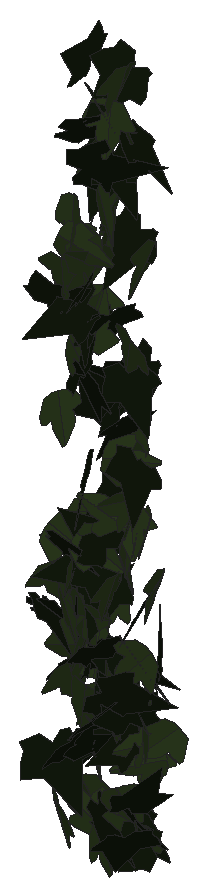
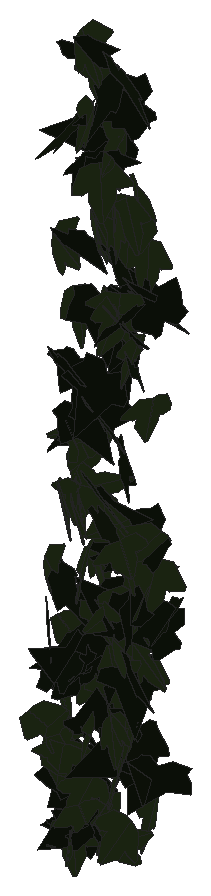
# SketchUp Ruby script. Lengths in inches.
U = 1.inch
M = Sketchup.active_model
def pt(a) = Geom::Point3d.new(a.map { |v| v * U })
def face(e, loops, mat)
  f = e.add_face(loops[0].map { |a| pt(a) })
  loops[1..].each { |l| e.add_face(l.map { |a| pt(a) }).erase! }
  f.material = f.back_material = mat if mat
  f
end
# faces: each face lists its corners as indices into pts; further lists are holes
def faces(e, pts, list, mat = nil) = list.each { |f| face(e, (f[0].is_a?(Array) ? f : [f]).map { |l| l.map { |i| pts[i] } }, mat) }
# xy, xz, yz: faces in a plane at the given z, y or x. An outline is a flat list of corners, or four numbers for a rectangle; further outlines are holes
def ring(l) = l.size == 4 ? [[l[0], l[1]], [l[2], l[1]], [l[2], l[3]], [l[0], l[3]]] : l.each_slice(2).to_a
def flat(e, list, mat, &to3) = list.each { |f| face(e, (f[0].is_a?(Array) ? f : [f]).map { |l| ring(l).map { |u, v| to3.(u, v) } }, mat) }
def xy(e, z, list, mat = nil) = flat(e, list, mat) { |x, y| [x, y, z] }
def xz(e, y, list, mat = nil) = flat(e, list, mat) { |x, z| [x, y, z] }
def yz(e, x, list, mat = nil) = flat(e, list, mat) { |y, z| [x, y, z] }
def lines(e, pts, list) = list.each { |a, b| e.add_line(pt(pts[a]), pt(pts[b])) }
# prism: a flat outline (further loops are holes) pulled along v
def prism(e, loops, v, mat = nil)
  f = face(e, loops, mat); d = Geom::Vector3d.new(v.map { |x| x * U })
  f.pushpull(f.normal.samedirection?(d) ? d.length : -d.length)
end
def box(e, o, s, mat = nil) = prism(e, [[o, [o[0] + s[0], o[1], o[2]], [o[0] + s[0], o[1] + s[1], o[2]], [o[0], o[1] + s[1], o[2]]]], [0, 0, s[2]], mat)
def at(x, y, z, deg = 0) = Geom::Transformation.translation(pt([x, y, z])) * Geom::Transformation.rotation(ORIGIN, Z_AXIS, deg.degrees)
def axes(o, x, y, z) = Geom::Transformation.new([*x, 0, *y, 0, *z, 0, *pt(o).to_a, 1])
def part(name) = M.definitions.add(name)
# library, detail: a bought-in or finely detailed component or shape, given as its bounding box
def library(name, o, s) = part(name).tap { |d| box(d.entities, o, s) }
def detail(e, o, s) = box(e.add_group.entities, o, s)
def put(e, d, t, mat = nil) = e.add_instance(d, t).tap { |i| i.material = mat if mat }
def group(e, t, mat = nil) = e.add_group.tap { |g| g.transformation = t; g.material = mat if mat }.entities
root = M.entities
M.materials.add("efeu1").color = [18, 25, 13]
M.materials.add("efeu2").color = [43, 57, 29]
c1 = part("ivyleaf_10")
p = [[0,0.5,-0.03],[-0.0625,2.02,-0.43],[-0.19,2.01,-0.46],[-0.54,1.05,-0.29],[-0.52,0.625,-0.18],[-0.83,0.76,-0.28],
  [-1.16,0.64,-0.33],[-1.15,0.33,-0.24],[-0.77,-0.39,0.02],[-0.3,-0.51,0.16],[0.04,-0.48,0.23],[-0.02,2.01,-0.4375],
  [-0.06,2.01,-0.43],[0.04,-0.49,0.23],[0.67,-0.49,0.14],[1.38,0.36,-0.2],[1.375,0.51,-0.24],[0.81,0.65,-0.19],
  [0.62,0.59,-0.15],[0.6,1.09,-0.28],[0.5,1.23,-0.31]]
faces(c1.entities,p,[[0,1,2,3,4,5,6,7,8,9,10],[11,12,0,13,14,15,16,17,18,19,20]],"efeu2")
c2 = part("ivyleaf_9")
p = [[1.54,2.16,1.25],[1.36,2.04,1.19],[-0.21,0.99,0.68],[-0.71,1.11,0.82],[-0.85,0.86,0.67],[-0.8,0.17,0.21],
  [-0.9,-0.01,0.1],[-0.67,-0.16,-0.02],[-0.08,-0.08,-0.05],[-0.03,-0.6,-0.4],[0.65,-0.88,-0.66],[0.83,-0.6,-0.49],
  [1.29,-0.42,-0.43],[1.8125,-0.07,-0.26],[1.21,0.44,0.15]]
faces(c2.entities,p,[[0,1,2,3,4,5,6,7,8,9,10,11,12,13,14]],"efeu1")
put(root,c1,axes([596.16,130.73,236.16],[0.80114,-0.40571,0.31651],[0.30205,-0.10337,-0.89704],[0.41658,0.85517,0.04172]))
put(root,c1,axes([597.11,131.1875,233.47],[-0.43594,-0.46998,-0.78449],[-0.3334,-0.72757,0.62115],[-0.85156,0.52546,0.15841]))
put(root,c2,axes([599.37,130.28,207.83],[0.2307,0.86352,-0.3889],[-0.20134,-0.3464,-0.88859],[-0.9254,0.29064,0.09638]))
put(root,c1,axes([596.39,130.43,234.79],[-0.41845,0.00511,-0.92472],[0.92464,-0.01195,-0.41848],[-0.01299,-1.01492,0.00027]))
put(root,c2,axes([597.37,130.25,228.79],[0.77939,0.02062,-0.64117],[-0.64046,-0.0325,-0.77957],[-0.03657,1.00871,-0.01201]))
put(root,c2,axes([594.78,130.71,217.05],[0.53253,-0.66296,0.09256],[0.08868,-0.04736,-0.84945],[0.66349,0.53843,0.03925]))
put(root,c2,axes([595.66,130.33,220.5],[0.97887,-0.06898,0.12471],[0.12456,-0.00655,-0.9813],[0.06926,0.98676,0.0022]))
put(root,c1,axes([595.9,130.35,208.03],[-0.78083,0.60175,0.16888],[-0.12797,0.1106,-0.98575],[-0.61175,-0.79119,-0.00935]))
put(root,c1,axes([596.02,130.51,233.42],[-0.91923,-0.11286,0.1591],[-0.16028,0.0002,-0.92593],[0.11118,-0.9329,-0.01945]))
put(root,c1,axes([598.875,131.33,223.06],[-0.11125,-0.17882,-0.91596],[-0.32327,-0.85796,0.20676],[-0.87548,0.33952,0.04005]))
put(root,c2,axes([596.7,130.97,231.61],[-1.02337,0.02852,0.26005],[-0.26032,-0.00706,-1.02367],[-0.02591,-1.05587,0.01387]))
put(root,c2,axes([597.9,130.08,212.98],[0.05111,0.96688,0.22476],[-0.13214,0.22968,-0.95801],[-0.98383,0.01938,0.14035]))
put(root,c1,axes([598.23,130.89,219.17],[0.12401,-0.92503,0.0834],[0.00161,-0.08393,-0.93326],[0.92878,0.12365,-0.00952]))
put(root,c1,axes([596.875,130.74,235.18],[-0.87155,0.03602,0.36956],[-0.37007,-0.16135,-0.85702],[0.03035,-0.93282,0.16251]))
put(root,c1,axes([595.9,131.4375,219.11],[0.09444,-0.17868,0.97324],[0.59515,-0.7708,-0.19927],[0.79051,0.60165,0.03375]))
put(root,c2,axes([597.98,130.65,220.9],[-0.25243,0.27697,0.87213],[-0.76993,0.42462,-0.3577],[-0.4945,-0.80252,0.11173]))
put(root,c1,axes([598.05,130.86,241.17],[0.98959,0.09097,0.06116],[0.05395,0.07936,-0.99101],[-0.09543,0.9883,0.07394]))
put(root,c1,axes([595.5,130.67,219.01],[-0.6191,-0.77198,-0.28301],[0.1729,0.22412,-0.98955],[0.80384,-0.64276,-0.00513]))
put(root,c1,axes([595.91,130.67,217.84],[-0.50003,0.94653,0.04891],[-0.01789,0.04586,-1.07047],[-0.94762,-0.50032,-0.00559]))
put(root,c2,axes([598.9,131.12,212.85],[0.52454,0.20871,0.81274],[-0.81511,-0.10086,0.55197],[0.19925,-0.96204,0.11845]))
put(root,c2,axes([596.65,131.32,224.0625],[-0.42628,0.09124,-0.85782],[0.79312,-0.33489,-0.42975],[-0.3393,-0.89744,0.07316]))
put(root,c2,axes([598.35,130.27,214.29],[0.16464,0.2909,-0.99963],[0.3502,0.9376,0.33053],[0.98043,-0.38376,0.0498]))
put(root,c2,axes([594.81,131.03,231.03],[-0.03401,-0.21356,0.95677],[0.87202,-0.44398,-0.0681],[0.44788,0.8482,0.20525]))
put(root,c2,axes([596.4375,130.4,211.31],[-0.07577,1.08266,0.05384],[-0.01537,0.0529,-1.08525],[-1.08389,-0.07644,0.01162]))
put(root,c1,axes([595.52,130.83,226.7],[0.33173,0.8446,0.03987],[0.01331,0.03761,-0.90741],[-0.84544,0.33199,0.00136]))
put(root,c1,axes([597.04,130.66,220.79],[0.43299,0.25024,0.81071],[0.68775,0.4295,-0.49989],[-0.49686,0.81257,0.01456]))
put(root,c1,axes([598.37,131.09,222.02],[0.37679,0.34332,0.82398],[-0.73129,-0.39416,0.49864],[0.51189,-0.81582,0.10584]))
put(root,c2,axes([597,131.01,233.11],[-0.67267,0.60958,-0.30603],[0.24231,-0.18822,-0.90752],[-0.63759,-0.71465,-0.02202]))
put(root,c2,axes([597.16,130.46,238.36],[0.6165,0.11599,0.96774],[0.94982,0.18537,-0.62731],[-0.21863,1.13235,0.00356]))
put(root,c1,axes([596.1,130.79,214.48],[-0.33067,-0.91612,-0.35897],[0.11507,0.34009,-0.97394],[0.97718,-0.35005,-0.00678]))
put(root,c2,axes([596.45,130.39,239.97],[0.73422,0.24002,0.58467],[0.47893,0.37349,-0.75476],[-0.4124,0.86106,0.16441]))
put(root,c1,axes([597.72,130.88,236.98],[-0.39079,0.89199,-0.03382],[0.01879,-0.02869,-0.97383],[-0.89244,-0.3912,-0.00569]))
put(root,c2,axes([599.01,131.52,224.75],[-0.01816,-0.95704,0.09186],[-0.00604,-0.09176,-0.95721],[0.96142,-0.01865,-0.00428]))
put(root,c1,axes([597.83,130.74,207.46],[-0.03252,1.02405,0.21124],[-0.13303,0.20557,-1.01705],[-1.03711,-0.05848,0.12383]))
put(root,c2,axes([597.37,131.51,219.52],[-0.83215,-0.05968,0.62281],[-0.59393,-0.25048,-0.81757],[0.19671,-1.00877,0.16616]))
put(root,c1,axes([596.3125,131.17,216.79],[-0.36918,-0.06357,0.93024],[0.93183,0.00994,0.37049],[-0.03271,1.00077,0.0554]))
put(root,c1,axes([596.84,130.96,213.48],[-1.01203,-0.03048,0.33589],[-0.33545,-0.01922,-1.01245],[0.03498,-1.06614,0.00865]))
put(root,c2,axes([595.02,131.06,210.35],[-0.3032,-0.64679,-0.80667],[0.39067,0.70665,-0.71344],[0.9573,-0.49324,0.03566]))
put(root,c2,axes([594.45,130.89,216.7],[0.66444,-0.15363,0.51724],[0.53596,0.09304,-0.66085],[0.06239,0.83688,0.16843]))
put(root,c1,axes([598.29,131.47,242.7],[0.07788,-1.01576,0.19504],[0.042,-0.19232,-1.0184],[1.03347,0.08436,0.02669]))
put(root,c2,axes([597.45,131.11,208.24],[0.71715,-0.65764,-0.35551],[-0.23436,0.27004,-0.97229],[0.7099,0.75351,0.03816]))
put(root,c1,axes([599.11,131.07,230.47],[-0.80845,0.21956,0.49643],[-0.47846,0.13238,-0.83773],[-0.25637,-0.93942,-0.00203]))
put(root,c2,axes([598.9,131.27,208.79],[0.67129,0.69571,0.17028],[-0.12472,-0.11627,0.96673],[0.7053,-0.68272,0.00888]))
put(root,c1,axes([595.44,130.85,220.63],[0.29673,0.63575,0.71383],[0.32066,0.63792,-0.70144],[-0.90051,0.43665,-0.01456]))
put(root,c1,axes([595.93,131.22,215.34],[-0.3503,0.11795,0.91701],[-0.92327,0.00722,-0.35362],[-0.04888,-0.98161,0.10758]))
put(root,c2,axes([596.73,130.66,228.56],[-0.03823,0.42167,0.97575],[-0.27142,0.94014,-0.41691],[-1.02772,-0.26398,0.07382]))
put(root,c1,axes([597.73,131.33,214.24],[-0.81731,0.56001,0.17259],[-0.29482,-0.13697,-0.95169],[-0.50644,-0.82403,0.27548]))
put(root,c1,axes([596.18,131.98,216],[0.29473,-0.66877,0.64401],[0.2584,-0.5899,-0.73083],[0.89176,0.39197,-0.00108]))
put(root,c1,axes([597.95,131,217.89],[-0.06514,0.27241,0.89044],[-0.77235,0.48281,-0.2042],[-0.52015,-0.75101,0.1917]))
put(root,c2,axes([597.19,131.11,215.64],[0.287,0.87565,-0.16655],[-0.07633,-0.15018,-0.92114],[-0.88808,0.2959,0.02535]))
put(root,c1,axes([598.64,131.76,221.26],[0.65703,-0.60895,0.23322],[0.18396,-0.14453,-0.89564],[0.6256,0.68205,0.01844]))
put(root,c1,axes([599.25,131.52,215.6875],[0.77189,-0.09258,-0.62262],[-0.60479,0.16407,-0.77417],[0.17452,0.97803,0.07094]))
put(root,c1,axes([598.17,131.12,224.9],[-0.10191,-0.16946,-0.90765],[0.79772,0.44367,-0.1724],[0.46495,-0.79835,0.09685]))
put(root,c1,axes([596.05,131.13,229.41],[-0.17708,0.81153,0.39111],[-0.14253,0.36833,-0.82881],[-0.88951,-0.22058,0.05495]))
put(root,c1,axes([596.79,131.43,230.02],[0.99514,-0.27811,-0.08585],[0.09367,0.01645,1.03246],[-0.27558,-0.9987,0.04092]))
put(root,c2,axes([598.28,132.05,242.78],[-0.92097,-0.39666,0.0533],[-0.04957,-0.01966,-1.00276],[0.39715,-0.9223,-0.00155]))
put(root,c1,axes([598.49,131.65,222.07],[0.86641,0.20621,0.23006],[0.22143,0.06321,-0.89056],[-0.21545,0.8942,0.0099]))
put(root,c2,axes([597.04,132.09,218.41],[-0.53997,-0.74652,-0.13099],[0.08202,0.10233,-0.92131],[0.75347,-0.54613,0.00642]))
put(root,c1,axes([598.64,131.59,222.33],[0.43867,-0.7577,-0.29504],[-0.12071,0.27084,-0.87502],[0.8041,0.45401,0.0296]))
put(root,c1,axes([597.92,131.875,213.8125],[-0.00733,0.0213,-0.94912],[0.85433,-0.41376,-0.01588],[-0.414,-0.85421,-0.01597]))
put(root,c2,axes([596.97,131.36,241.16],[0.83223,-0.15985,-0.48672],[-0.46453,0.15604,-0.84553],[0.21602,0.9514,0.0569]))
put(root,c2,axes([596.09,131.23,214.78],[0.07354,1.04441,-0.04536],[-0.06908,-0.04052,-1.04491],[-1.04311,0.07631,0.066]))
put(root,c2,axes([597.61,131.45,231.18],[0.1594,0.87779,-0.31583],[-0.10034,-0.30242,-0.89115],[-0.92747,0.18358,0.04213]))
put(root,c2,axes([596.13,132.22,230.84],[-0.05738,-0.91352,0.11727],[-0.02367,-0.116,-0.91518],[0.92071,-0.05991,-0.01622]))
put(root,c1,axes([596.4,131.7,231.5625],[0.73465,0.60201,0.14105],[0.11793,0.0786,-0.9497],[-0.60696,0.74393,-0.0138]))
put(root,c2,axes([598.43,131.86,211.37],[-0.81989,0.324,0.15755],[-0.15175,0.04463,-0.88148],[-0.32676,-0.8337,0.01405]))
put(root,c2,axes([597.33,131.79,221.375],[-0.69004,0.61843,-0.06955],[0.04704,-0.05171,-0.92658],[-0.62054,-0.6916,0.00709]))
put(root,c2,axes([596.31,131.13,210.81],[0.58304,0.47403,0.66189],[0.51765,0.4125,-0.75141],[-0.62836,0.77966,-0.00487]))
put(root,c2,axes([599.05,132.14,206.65],[-0.47623,-0.46464,-0.5611],[-0.3847,-0.40887,0.66509],[-0.61865,0.61193,0.01835]))
put(root,c2,axes([597.42,132.52,214.57],[-0.34965,-0.78655,0.29494],[-0.11445,-0.27189,-0.86075],[0.8322,-0.36786,0.00555]))
put(root,c1,axes([598.04,131.73,208.81],[-0.75663,-0.34763,-0.33872],[0.30448,0.14858,-0.83263],[0.37798,-0.81556,-0.00731]))
put(root,c1,axes([599.2,131.92,221.83],[0.53142,-0.7488,-0.1849],[-0.08168,0.16864,-0.91771],[0.76696,0.5368,0.03038]))
put(root,c2,axes([596.74,131.52,230.32],[-0.23803,0.54178,0.76344],[-0.60639,0.5109,-0.55163],[-0.7132,-0.6152,0.21422]))
put(root,c2,axes([596.99,132.28,226.375],[0.50327,0.16234,0.84395],[-0.80768,-0.24489,0.52874],[0.29371,-0.95161,0.00791]))
put(root,c2,axes([597.02,132.39,238.11],[-0.61915,-0.71721,-0.14046],[0.10834,0.09198,-0.94724],[0.72276,-0.62818,0.02167]))
put(root,c1,axes([596.48,131.7,231.11],[-0.48545,-0.7056,-0.43436],[0.24009,0.36204,-0.85644],[0.79303,-0.54153,-0.00661]))
put(root,c1,axes([599.42,131.44,212.37],[0.32256,-0.132,-0.88914],[-0.47315,0.77827,-0.28718],[0.76428,0.53751,0.19746]))
put(root,c1,axes([596.8125,131.28,238.49],[0.13973,0.24038,0.92181],[-0.48352,0.82064,-0.1407],[-0.8208,-0.4425,0.23981]))
put(root,c2,axes([598.17,132.09,228.39],[-0.37118,-0.47083,-0.70904],[0.55568,0.45188,-0.59095],[0.64471,-0.66055,0.10113]))
put(root,c1,axes([598.9,132.59,211.125],[-0.08428,0.13445,0.85306],[-0.13602,-0.84848,0.12029],[0.85281,-0.12205,0.10349]))
put(root,c1,axes([596.28,132.24,212.62],[0.82567,-0.34136,0.33469],[0.30266,-0.14381,-0.89331],[0.37007,0.87924,-0.01616]))
put(root,c2,axes([599.09,132.17,218.19],[-0.53979,0.56241,-0.45279],[0.30054,-0.33901,-0.77938],[-0.6565,-0.61762,0.0155]))
put(root,c2,axes([598.19,132.13,226.19],[-0.22635,0.71247,-0.5332],[-0.03355,-0.55662,-0.72952],[-0.88926,-0.16035,0.16324]))
put(root,c1,axes([599.14,132.55,210.39],[-0.14162,-0.06921,0.89006],[-0.52855,-0.71976,-0.14007],[0.71946,-0.5424,0.0723]))
put(root,c1,axes([596.22,132.15,206.93],[0.4931,0.20575,0.77948],[-0.73194,-0.26873,0.53397],[0.33791,-0.88234,0.01914]))
put(root,c2,axes([596.12,131.79,214.96],[-0.30769,0.03101,-0.92375],[-0.92426,-0.01549,0.30734],[-0.0049,0.97352,0.03431]))
put(root,c1,axes([596.21,131.67,217.77],[-0.34469,-0.41366,-0.79733],[0.57601,0.55352,-0.53618],[0.68925,-0.66945,0.04934]))
put(root,c2,axes([597.49,132.28,223.07],[-0.89004,0.34188,-0.12334],[0.11186,-0.05275,-0.9534],[-0.3458,-0.897,0.00906]))
put(root,c1,axes([596.41,132.19,212.27],[0.00463,-0.84912,-0.08516],[0.01124,0.08521,-0.84905],[0.8533,0.00349,0.01165]))
put(root,c2,axes([595.98,131.95,217.07],[-0.17476,-0.09602,0.92837],[0.93332,-0.01938,0.17369],[0.00139,0.94447,0.09795]))
put(root,c1,axes([595.43,132.05,212.73],[-0.63582,0.74131,-0.05731],[0.03739,-0.04343,-0.97663],[-0.74258,-0.63692,-0.00011]))
put(root,c2,axes([597.27,132.28,238.26],[0.16703,-0.85602,-0.40201],[-0.05635,0.3985,-0.87196],[0.94404,0.17525,0.01908]))
put(root,c1,axes([599.24,132.62,218.9],[0.2989,-0.74313,0.42144],[0.18761,-0.37849,-0.80046],[0.83346,0.3517,0.02905]))
put(root,c1,axes([596.78,132.58,235.22],[0.63729,-0.45419,0.59866],[0.52172,-0.2975,-0.7811],[0.54082,0.8222,0.04808]))
put(root,c1,axes([598.63,132.73,233.97],[0.2476,-0.77973,0.55458],[0.18285,-0.52374,-0.81799],[0.9392,0.30752,0.01305]))
put(root,c2,axes([597.64,132.25,207.49],[0.65729,-0.28132,0.44555],[0.40021,-0.19684,-0.71468],[0.34276,0.76929,-0.01993]))
put(root,c1,axes([596.45,131.92,214.26],[0.48998,0.78036,-0.26153],[0.14738,0.21626,0.92138],[0.80972,-0.51157,-0.00944]))
put(root,c2,axes([595.89,131.65,216.93],[0.00155,-0.14848,0.98461],[0.0975,0.97991,0.14762],[-0.99096,0.09618,0.01607]))
put(root,c1,axes([597.47,131.98,212.3],[-0.36657,0.77591,0.31223],[-0.13028,0.28377,-0.85813],[-0.82617,-0.38902,-0.00321]))
put(root,c1,axes([597.09,132.41,217.5],[0.82688,-0.06508,-0.29164],[-0.29036,0.02777,-0.82942],[0.07061,0.87637,0.00462]))
put(root,c2,axes([597.6,132.05,226.58],[-0.5518,0.63144,0.38447],[-0.28499,0.26099,-0.83767],[-0.68215,-0.61983,0.03896]))
put(root,c1,axes([596.16,132.17,210.29],[-0.52956,0.65109,0.03916],[-0.02469,0.0304,-0.83926],[-0.6518,-0.53014,-0.00002]))
put(root,c2,axes([598.65,132.86,214.03],[0.8073,-0.80675,0.17196],[-0.11658,0.1266,1.14129],[-0.8166,-0.81565,0.00707]))
put(root,c1,axes([596.91,132.6,235.46],[0.44273,-0.8795,0.1597],[0.09008,-0.13341,-0.98444],[0.88933,0.45135,0.02021]))
put(root,c1,axes([597.56,132.34,239.93],[-0.67804,0.68925,-0.21859],[0.13403,-0.17466,-0.9665],[-0.71055,-0.69067,0.02628]))
put(root,c2,axes([597.46,132.1875,211.96],[-0.67613,-0.43593,0.43437],[0.36056,0.24235,0.80445],[-0.49871,0.76623,-0.00731]))
put(root,c1,axes([598.4,132.4,206.9],[-0.92213,-0.11223,0.20381],[-0.18412,-0.15731,-0.91968],[0.14225,-0.93119,0.1308]))
put(root,c1,axes([597.73,132.51,208.08],[0.57458,0.62679,-0.25093],[-0.17293,-0.18187,-0.85029],[-0.65263,0.60003,0.00439]))
put(root,c1,axes([597.93,132.85,224.99],[0.04375,-0.15808,-0.89931],[0.58646,-0.68523,0.14898],[-0.69987,-0.58407,0.06862]))
put(root,c1,axes([596.89,132.4375,237.46],[-0.74391,-0.5883,0.10521],[-0.08392,-0.06349,-0.94841],[0.59171,-0.74862,-0.00224]))
put(root,c1,axes([597.88,132.11,219.44],[-0.54431,0.64498,0.34261],[-0.23684,0.24832,-0.84374],[-0.69086,-0.59329,0.01931]))
put(root,c2,axes([598.05,132.43,239.42],[0.65299,-0.71391,-0.19548],[-0.01939,0.24409,-0.9562],[0.73993,0.63641,0.14745]))
put(root,c1,axes([595.59,132.625,220.97],[0.48038,0.74854,-0.25402],[-0.11896,-0.22541,-0.88918],[-0.78146,0.49445,-0.0208]))
put(root,c1,axes([596.32,132.07,235.59],[0.23747,-0.57909,-0.77378],[-0.30313,0.71196,-0.62585],[0.91771,0.38502,-0.0065]))
put(root,c1,axes([599.76,132.74,211.8],[0.54862,0.24639,-0.65135],[-0.6379,-0.15483,-0.59586],[-0.27936,0.83741,0.08147]))
put(root,c2,axes([597.86,132.4,207.32],[-0.06626,-0.17685,-0.82213],[0.53383,0.62836,-0.17819],[0.64977,-0.53428,0.06256]))
put(root,c1,axes([598.66,132.53,210.49],[0.7628,0.41804,0.17335],[0.14197,0.10154,-0.8696],[-0.42971,0.77563,0.02042]))
put(root,c2,axes([597.78,132.77,214.44],[0.46824,-0.39976,0.7706],[0.65977,-0.40518,-0.61108],[0.56422,0.80555,0.07506]))
put(root,c2,axes([597.91,132.99,234.57],[-0.8838,-0.3506,-0.16234],[0.16661,0.01982,-0.94985],[0.34859,-0.89837,0.0424]))
put(root,c2,axes([596.84,132.15,228.14],[0.72254,0.58524,-0.09618],[-0.07531,-0.05983,-0.92982],[-0.58829,0.72645,0.00091]))
put(root,c1,axes([598.42,132.16,207.07],[0.25958,-0.47404,-0.71017],[-0.15402,0.70409,-0.52628],[0.83984,0.27564,0.12298]))
put(root,c2,axes([595.97,132.23,242.38],[-0.51041,0.73188,0.45878],[-0.29321,0.35446,-0.89165],[-0.8125,-0.58767,0.03356]))
put(root,c2,axes([599.67,132.19,215.1875],[0.07954,-0.15827,0.8892],[-0.10108,0.88547,0.16664],[-0.8975,-0.11376,0.06003]))
put(root,c2,axes([598.47,132.92,228.62],[-0.88133,0.06809,-0.30179],[0.30181,-0.01103,-0.88388],[-0.068,-0.9315,-0.01159]))
put(root,c1,axes([595.55,132.62,208.05],[-0.89119,0.16498,-0.40078],[0.39277,-0.08001,-0.90631],[-0.18324,-0.97388,0.00657]))
